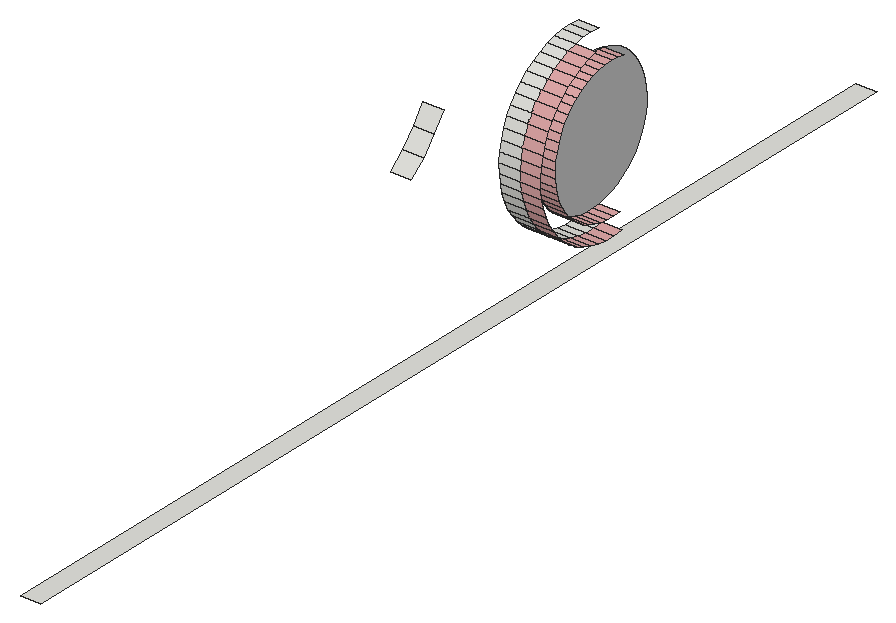
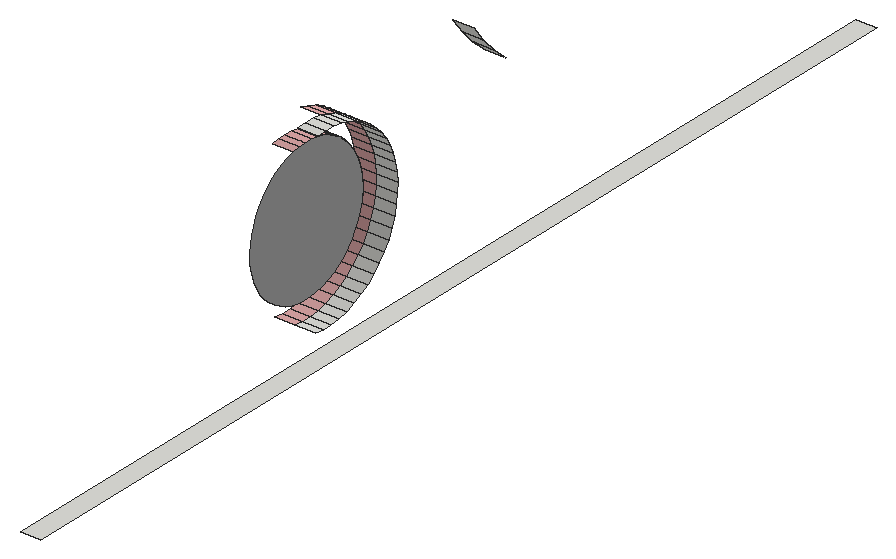
# SketchUp Ruby script. Lengths in inches.
U = 1.inch
M = Sketchup.active_model
def pt(a) = Geom::Point3d.new(a.map { |v| v * U })
def face(e, loops, mat)
  f = e.add_face(loops[0].map { |a| pt(a) })
  loops[1..].each { |l| e.add_face(l.map { |a| pt(a) }).erase! }
  f.material = f.back_material = mat if mat
  f
end
# faces: each face lists its corners as indices into pts; further lists are holes
def faces(e, pts, list, mat = nil) = list.each { |f| face(e, (f[0].is_a?(Array) ? f : [f]).map { |l| l.map { |i| pts[i] } }, mat) }
# xy, xz, yz: faces in a plane at the given z, y or x. An outline is a flat list of corners, or four numbers for a rectangle; further outlines are holes
def ring(l) = l.size == 4 ? [[l[0], l[1]], [l[2], l[1]], [l[2], l[3]], [l[0], l[3]]] : l.each_slice(2).to_a
def flat(e, list, mat, &to3) = list.each { |f| face(e, (f[0].is_a?(Array) ? f : [f]).map { |l| ring(l).map { |u, v| to3.(u, v) } }, mat) }
def xy(e, z, list, mat = nil) = flat(e, list, mat) { |x, y| [x, y, z] }
def xz(e, y, list, mat = nil) = flat(e, list, mat) { |x, z| [x, y, z] }
def yz(e, x, list, mat = nil) = flat(e, list, mat) { |y, z| [x, y, z] }
def lines(e, pts, list) = list.each { |a, b| e.add_line(pt(pts[a]), pt(pts[b])) }
# prism: a flat outline (further loops are holes) pulled along v
def prism(e, loops, v, mat = nil)
  f = face(e, loops, mat); d = Geom::Vector3d.new(v.map { |x| x * U })
  f.pushpull(f.normal.samedirection?(d) ? d.length : -d.length)
end
def box(e, o, s, mat = nil) = prism(e, [[o, [o[0] + s[0], o[1], o[2]], [o[0] + s[0], o[1] + s[1], o[2]], [o[0], o[1] + s[1], o[2]]]], [0, 0, s[2]], mat)
def at(x, y, z, deg = 0) = Geom::Transformation.translation(pt([x, y, z])) * Geom::Transformation.rotation(ORIGIN, Z_AXIS, deg.degrees)
def axes(o, x, y, z) = Geom::Transformation.new([*x, 0, *y, 0, *z, 0, *pt(o).to_a, 1])
def part(name) = M.definitions.add(name)
# library, detail: a bought-in or finely detailed component or shape, given as its bounding box
def library(name, o, s) = part(name).tap { |d| box(d.entities, o, s) }
def detail(e, o, s) = box(e.add_group.entities, o, s)
def put(e, d, t, mat = nil) = e.add_instance(d, t).tap { |i| i.material = mat if mat }
def group(e, t, mat = nil) = e.add_group.tap { |g| g.transformation = t; g.material = mat if mat }.entities
root = M.entities
M.materials.add("Generic").color = [224, 169, 169]
M.materials.add("[Mirror 01]").color = [185, 185, 185]
xy(root,46.5,[[9,94.93,10.6875,181.21]])
xy(root,50.75,[[10.6875,151.32,12.375,151.96]],"Generic")
yz(root,10.6875,[[151.32,50.75,151.96,50.75,152.59,50.8125,153.22,50.95,153.83,51.15,154.41,51.42,154.96,51.75,155.47,52.14,155.93,52.58,156.34,53.07,156.7,53.6,156.99,54.17,157.22,54.77,157.38,55.39,157.48,56.02,157.5,56.66,157.45,57.3,157.34,57.93,157.15,58.54,156.9,59.13,156.58,59.6875,156.21,60.21,155.78,60.68,155.3,61.11,154.78,61.48,154.22,61.79,153.63,62.04,153.01,62.22,152.38,62.33,151.74,62.37,151.1,62.34,150.47,62.24,149.85,62.07,149.26,61.83,148.69,61.54,148.16,61.18,147.68,60.76,147.24,60.29,146.85,59.78,146.53,59.23,146.27,58.64,146.07,58.03,145.94,57.41,145.88,56.77,145.89,56.13,145.97,55.49,146.125,54.87,146.35,54.27,146.63,53.7,146.97,53.16,147.375,52.66,147.83,52.21,148.33,51.81,148.875,51.47,149.45,51.19,150.06,50.98,150.68,50.83]],"[Mirror 01]")
p = [[10.6875,150.42,49.36],[10.6875,151.22,49.26],[9,151.22,49.26],[9,150.42,49.36],[12.375,151.22,49.26],[12.375,150.42,49.36],
  [10.6875,152.02,49.25],[9,152.02,49.25],[12.375,152.02,49.25],[10.6875,152.83,49.33],[9,152.83,49.33],[12.375,152.83,49.33],
  [10.6875,149.63,49.54],[9,149.63,49.54],[12.375,149.63,49.54],[10.6875,148.875,49.81],[9,148.875,49.81],[12.375,148.875,49.81],
  [10.6875,148.15,50.16],[9,148.15,50.16],[12.375,148.15,50.16],[10.6875,147.47,50.59],[9,147.47,50.59],[12.375,147.47,50.59],
  [10.6875,146.84,51.09],[9,146.84,51.09],[12.375,146.84,51.09],[10.6875,152.59,50.8125],[10.6875,151.96,50.75],[12.375,151.96,50.75],
  [12.375,152.59,50.8125],[10.6875,150.68,50.83],[10.6875,150.06,50.98],[12.375,150.06,50.98],[12.375,150.68,50.83],[10.6875,151.32,50.75],
  [12.375,151.32,50.75],[10.6875,149.45,51.19],[12.375,149.45,51.19],[10.6875,146.26,51.65],[9,146.26,51.65],[12.375,146.26,51.65],
  [10.6875,148.875,51.47],[12.375,148.875,51.47],[10.6875,148.33,51.81],[12.375,148.33,51.81],[10.6875,145.76,52.28],[9,145.76,52.28],
  [12.375,145.76,52.28],[10.6875,147.83,52.21],[12.375,147.83,52.21],[10.6875,147.375,52.66],[12.375,147.375,52.66],[10.6875,145.32,52.96],
  [9,145.32,52.96],[12.375,145.32,52.96],[10.6875,146.97,53.16],[12.375,146.97,53.16],[10.6875,144.97,53.68],[9,144.97,53.68],
  [12.375,144.97,53.68],[10.6875,146.63,53.7],[12.375,146.63,53.7],[10.6875,144.69,54.4375],[9,144.69,54.4375],[12.375,144.69,54.4375],
  [10.6875,146.35,54.27],[12.375,146.35,54.27],[10.6875,146.125,54.87],[12.375,146.125,54.87],[10.6875,144.5,55.22],[9,144.5,55.22],
  [12.375,144.5,55.22],[10.6875,145.97,55.49],[12.375,145.97,55.49],[10.6875,144.4,56.02],[9,144.4,56.02],[12.375,144.4,56.02],
  [10.6875,145.89,56.13],[12.375,145.89,56.13],[10.6875,144.38,56.82],[9,144.38,56.82],[12.375,144.38,56.82],[10.6875,145.88,56.77],
  [12.375,145.88,56.77],[10.6875,144.46,57.625],[9,144.46,57.625],[12.375,144.46,57.625],[10.6875,145.94,57.41],[12.375,145.94,57.41],
  [10.6875,146.07,58.03],[12.375,146.07,58.03],[10.6875,144.62,58.42],[9,144.62,58.42],[12.375,144.62,58.42],[10.6875,146.27,58.64],
  [12.375,146.27,58.64],[10.6875,144.87,59.18],[9,144.87,59.18],[12.375,144.87,59.18],[10.6875,146.53,59.23],[12.375,146.53,59.23],
  [10.6875,145.2,59.92],[9,145.2,59.92],[12.375,145.2,59.92],[10.6875,146.85,59.78],[12.375,146.85,59.78],[10.6875,147.24,60.29],
  [12.375,147.24,60.29],[10.6875,145.61,60.61],[9,145.61,60.61],[12.375,145.61,60.61],[10.6875,147.68,60.76],[12.375,147.68,60.76],
  [10.6875,146.09,61.26],[9,146.09,61.26],[12.375,146.09,61.26],[10.6875,148.16,61.18],[12.375,148.16,61.18],[10.6875,133.17,61.09],
  [10.6875,134.4375,62.1875],[9,134.4375,62.1875],[9,133.17,61.09],[10.6875,148.69,61.54],[12.375,148.69,61.54],[10.6875,146.64,61.84],
  [9,146.64,61.84],[12.375,146.64,61.84],[10.6875,149.26,61.83],[12.375,149.26,61.83],[10.6875,147.25,62.37],[9,147.25,62.37],
  [12.375,147.25,62.37],[10.6875,149.85,62.07],[12.375,149.85,62.07],[10.6875,150.47,62.24],[12.375,150.47,62.24],[10.6875,135.5625,63.42],
  [9,135.5625,63.42],[10.6875,151.1,62.34],[12.375,151.1,62.34],[10.6875,152.38,62.33],[10.6875,153.01,62.22],[12.375,153.01,62.22],
  [12.375,152.38,62.33],[10.6875,151.74,62.37],[12.375,151.74,62.37],[10.6875,147.92,62.82],[9,147.92,62.82],[12.375,147.92,62.82],
  [10.6875,148.63,63.2],[9,148.63,63.2],[12.375,148.63,63.2],[10.6875,149.38,63.49],[9,149.38,63.49],[12.375,149.38,63.49],
  [10.6875,136.54,64.77],[9,136.54,64.77],[10.6875,150.16,63.7],[9,150.16,63.7],[12.375,150.16,63.7],[10.6875,150.95,63.83],
  [9,150.95,63.83],[10.6875,151.76,63.87],[9,151.76,63.87],[10.6875,152.5625,63.81],[9,152.5625,63.81]]
faces(root,p,[[0,1,2,3],[1,6,7,2],[6,9,10,7],[12,0,3,13],[15,12,13,16],[18,15,16,19],[21,18,19,22],[24,21,22,25],
  [39,24,25,40],[46,39,40,47],[53,46,47,54],[58,53,54,59],[63,58,59,64],[70,63,64,71],[75,70,71,76],[80,75,76,81],
  [85,80,81,86],[92,85,86,93],[97,92,93,98],[102,97,98,103],[109,102,103,110],[114,109,110,115],[119,120,121,122],[125,114,115,126],
  [130,125,126,131],[120,137,138,121],[147,130,131,148],[150,147,148,151],[153,150,151,154],[137,156,157,138],[158,153,154,159],[161,158,159,162],
  [163,161,162,164],[165,163,164,166]])
faces(root,p,[[0,1,4,5],[1,6,8,4],[6,9,11,8],[12,0,5,14],[15,12,14,17],[18,15,17,20],[21,18,20,23],[24,21,23,26],
  [27,28,29,30],[31,32,33,34],[35,31,34,36],[32,37,38,33],[39,24,26,41],[37,42,43,38],[42,44,45,43],[46,39,41,48],
  [44,49,50,45],[49,51,52,50],[53,46,48,55],[51,56,57,52],[58,53,55,60],[56,61,62,57],[63,58,60,65],[61,66,67,62],
  [66,68,69,67],[70,63,65,72],[68,73,74,69],[75,70,72,77],[73,78,79,74],[80,75,77,82],[78,83,84,79],[85,80,82,87],
  [83,88,89,84],[88,90,91,89],[92,85,87,94],[90,95,96,91],[97,92,94,99],[95,100,101,96],[102,97,99,104],[100,105,106,101],
  [105,107,108,106],[109,102,104,111],[107,112,113,108],[114,109,111,116],[112,117,118,113],[117,123,124,118],[125,114,116,127],[123,128,129,124],
  [130,125,127,132],[128,133,134,129],[133,135,136,134],[135,139,140,136],[141,142,143,144],[139,145,146,140],[145,141,144,146],[147,130,132,149],
  [150,147,149,152],[153,150,152,155],[158,153,155,160]],"Generic")
